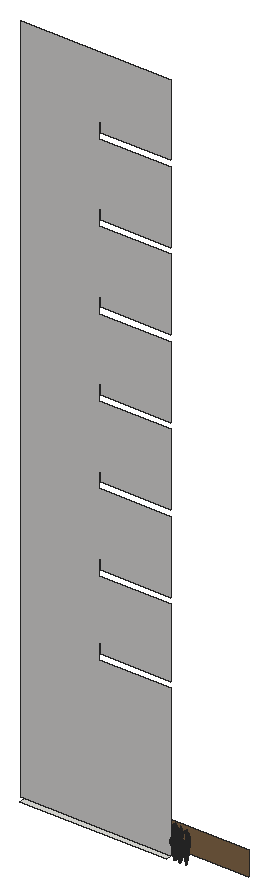
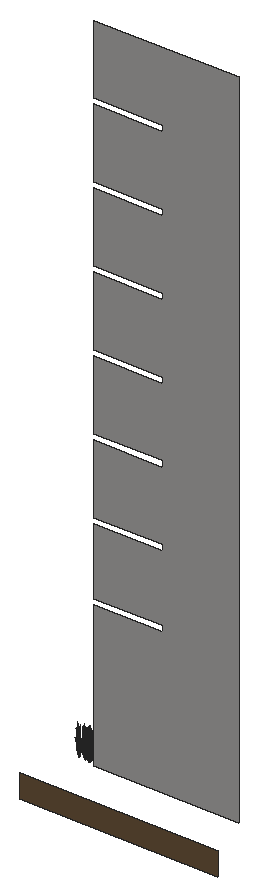
# SketchUp Ruby script. Lengths in inches.
U = 1.inch
M = Sketchup.active_model
def pt(a) = Geom::Point3d.new(a.map { |v| v * U })
def face(e, loops, mat)
  f = e.add_face(loops[0].map { |a| pt(a) })
  loops[1..].each { |l| e.add_face(l.map { |a| pt(a) }).erase! }
  f.material = f.back_material = mat if mat
  f
end
# faces: each face lists its corners as indices into pts; further lists are holes
def faces(e, pts, list, mat = nil) = list.each { |f| face(e, (f[0].is_a?(Array) ? f : [f]).map { |l| l.map { |i| pts[i] } }, mat) }
# xy, xz, yz: faces in a plane at the given z, y or x. An outline is a flat list of corners, or four numbers for a rectangle; further outlines are holes
def ring(l) = l.size == 4 ? [[l[0], l[1]], [l[2], l[1]], [l[2], l[3]], [l[0], l[3]]] : l.each_slice(2).to_a
def flat(e, list, mat, &to3) = list.each { |f| face(e, (f[0].is_a?(Array) ? f : [f]).map { |l| ring(l).map { |u, v| to3.(u, v) } }, mat) }
def xy(e, z, list, mat = nil) = flat(e, list, mat) { |x, y| [x, y, z] }
def xz(e, y, list, mat = nil) = flat(e, list, mat) { |x, z| [x, y, z] }
def yz(e, x, list, mat = nil) = flat(e, list, mat) { |y, z| [x, y, z] }
def lines(e, pts, list) = list.each { |a, b| e.add_line(pt(pts[a]), pt(pts[b])) }
# prism: a flat outline (further loops are holes) pulled along v
def prism(e, loops, v, mat = nil)
  f = face(e, loops, mat); d = Geom::Vector3d.new(v.map { |x| x * U })
  f.pushpull(f.normal.samedirection?(d) ? d.length : -d.length)
end
def box(e, o, s, mat = nil) = prism(e, [[o, [o[0] + s[0], o[1], o[2]], [o[0] + s[0], o[1] + s[1], o[2]], [o[0], o[1] + s[1], o[2]]]], [0, 0, s[2]], mat)
def at(x, y, z, deg = 0) = Geom::Transformation.translation(pt([x, y, z])) * Geom::Transformation.rotation(ORIGIN, Z_AXIS, deg.degrees)
def axes(o, x, y, z) = Geom::Transformation.new([*x, 0, *y, 0, *z, 0, *pt(o).to_a, 1])
def part(name) = M.definitions.add(name)
# library, detail: a bought-in or finely detailed component or shape, given as its bounding box
def library(name, o, s) = part(name).tap { |d| box(d.entities, o, s) }
def detail(e, o, s) = box(e.add_group.entities, o, s)
def put(e, d, t, mat = nil) = e.add_instance(d, t).tap { |i| i.material = mat if mat }
def group(e, t, mat = nil) = e.add_group.tap { |g| g.transformation = t; g.material = mat if mat }.entities
root = M.entities
M.materials.add("Carpet_01_1K").color = [196, 195, 193]
M.materials.add("LightPink_Translucent").color = [144, 107, 117]
M.materials["LightPink_Translucent"].alpha = 0.75
M.materials.add("Soil_03_1K").color = [122, 96, 67]
c1 = part("blade")
p = [[2.15,0.21,22],[0,0.17,0],[0.09,0.45,0],[2.18,0.31,22],[2.29,0.31,22],[0.38,0.45,0],
  [2.48,0.24,33],[2.49,0.24,33],[2.48,0.22,33]]
faces(c1.entities,p,[[0,1,2,3],[4,5,2,3],[6,3,4,7],[8,0,3,6]])
c2 = part("seeds")
p = [[0.3,-0.1,1.38],[-0.01,-0.03,1.59],[-0.01,-0.03,0.03],[0.14,-0.07,-0.07],[0.29,-0.03,3],[0.15,0.01,3.11]]
faces(c2.entities,p,[[0,1,2,3],[1,0,4,5]],"LightPink_Translucent")
c3 = part("blade with seeds")
put(c3.entities,c1,at(0,0,0))
put(c3.entities,c2,axes([2.4,0.25,30.99],[1.5799,-0.05474,1.17369],[-0.12525,1.92788,0.29478],[-0.07173,-0.02425,1.56792]))
xy(root,0,[[39.57,786.64,330.57,798.7]])
xz(root,798.7,[[30.57,0,30.57,1386,330.57,1386,330.57,1242,189.57,1242,189.57,1260,186.57,1260,186.57,1230,330.57,1230,330.57,1086,189.57,1086,189.57,1104,186.57,1104,186.57,1074,330.57,1074,330.57,930,189.57,930,189.57,948,186.57,948,186.57,918,330.57,918,330.57,774,189.57,774,189.57,791.9,186.57,791.9,186.57,762,330.57,762,330.57,618,189.57,618,189.57,636,186.57,636,186.57,606,330.57,606,330.57,462,189.57,462,189.57,480,186.57,480,186.57,450,330.57,450,330.57,312,189.57,312,189.57,330,186.57,330,186.57,300,330.57,300,330.57,0]],"Carpet_01_1K")
xz(root,890.67,[[0,-48,410.57,0]],"Soil_03_1K")
put(root,c3,axes([342.49,790.44,4.68],[-0.25628,0.30892,-0.51099],[-0.22444,-0.32634,-0.3958],[-0.13021,-0.047,0.97773]))
put(root,c3,axes([368.57,789.07,2.72],[0.38326,-0.02879,0.44739],[0.03466,0.47788,-0.21531],[-0.06861,0.04843,1.43643]))
put(root,c3,axes([368.8125,788.59,2.62],[0.32884,-0.136,0.1448],[0.11516,0.38837,-0.41347],[0,0.08547,1.26744]))
put(root,c3,axes([355.58,788.84,2.72],[0.17124,-0.42022,0.44739],[0.35581,0.20224,-0.21531],[0,0.09687,1.43643]))
put(root,c3,axes([341.92,790.85,2.77],[0.22533,-0.03337,1.1486],[-0.14293,0.29403,0.84392],[-0.11135,-0.04411,0.25299]))
put(root,c3,axes([368.23,789.3,2.21],[-0.38326,0.02879,-0.44739],[-0.03466,-0.47788,0.21531],[-0.06861,0.04843,1.43643]))
put(root,c3,axes([355.52,789.08,2.29],[0,0.53934,-0.05637],[-0.44133,0,0],[0,0.01695,1.79368]))
put(root,c3,axes([353.5,788.89,4.68],[-0.09562,0.42421,-0.51099],[-0.32782,-0.1454,-0.3958],[-0.13199,0.0389,0.97773]))
put(root,c3,axes([343.51,791.125,2.72],[-0.38326,0.02879,0.44739],[-0.03466,-0.47788,-0.21531],[0.06861,-0.04843,1.43643]))
put(root,c3,axes([355.55,788.7,2.21],[0.21202,0.39143,-0.44739],[-0.32115,0.27564,0.21531],[0.06861,0.04843,1.43643]))
put(root,c3,axes([356.99,790.36,3.93],[-0.06755,-0.39203,-0.03492],[0.31928,-0.09013,-0.15832],[0.06667,0.02485,0.52218]))
put(root,c3,axes([342.52,791.47,2.48],[0,0.46636,0.49651],[-0.39487,0,0],[0,-0.10622,1.57504]))
put(root,c3,axes([354.23,790.7,2.375],[-0.22066,0.46731,0],[-0.36918,-0.26061,-0.51607],[-0.08408,-0.05936,1.63711]))
put(root,c3,axes([345.29,791.58,4.68],[0.09562,-0.42421,-0.51099],[0.32782,0.1454,-0.3958],[0.13199,-0.0389,0.97773]))
put(root,c3,axes([344.77,789.85,2.375],[0.22066,-0.46731,0],[0.36918,0.26061,-0.51607],[0.08408,0.05936,1.63711]))
put(root,c3,axes([356.48,789.08,2.48],[0,-0.46636,0.49651],[0.39487,0,0],[0,0.10622,1.57504]))
put(root,c3,axes([342.17,790.77,3.875],[0.14639,-0.01056,1.71376],[-0.09712,0.45778,0.13857],[-0.20862,-0.02831,0.73262]))
put(root,c3,axes([368.52,789.95,2.2],[0.35581,0.20937,0],[-0.17124,0.43505,0],[0,0,1.74954]))
put(root,c3,axes([343.45,791.85,2.21],[-0.21202,-0.39143,-0.44739],[0.32115,-0.27564,0.21531],[-0.06861,-0.04843,1.43643]))
put(root,c3,axes([343.49,791.3,2.36],[0.15345,0.52148,0.45755],[-0.43845,0.18134,0.17955],[0.00536,-0.09582,1.58856]))
put(root,c3,axes([355.49,789.43,2.72],[0.38326,-0.02879,0.44739],[0.03466,0.47788,-0.21531],[-0.06861,0.04843,1.43643]))
put(root,c3,axes([355.73,788.9375,2.62],[0.32884,-0.136,0.1448],[0.11516,0.38837,-0.41347],[0,0.08547,1.26744]))
put(root,c3,axes([345.64,791.7,1.98],[-0.22732,0.05597,1.41583],[-0.03618,-0.44548,0.08104],[0.15921,-0.06743,0.80566]))
put(root,c3,axes([346.05,791.3,2.26],[-0.21881,-0.29821,-0.06488],[0.23965,-0.27324,-0.29416],[0.0679,-0.01924,0.97024]))
put(root,c3,axes([355.15,789.66,2.21],[-0.38326,0.02879,-0.44739],[-0.03466,-0.47788,0.21531],[-0.06861,0.04843,1.43643]))
put(root,c3,axes([368.66,790.41,2.19],[-0.21791,-0.46895,-0.05142],[0.36918,-0.26061,0.51607],[-0.09097,0.04465,1.6363]))
put(root,c3,axes([343.42,791.71,2.72],[-0.17124,0.42022,0.44739],[-0.35581,-0.20224,-0.21531],[0,-0.09687,1.43643]))
put(root,c3,axes([368.58,789.28,2.62],[0.26075,0.2802,0.1448],[-0.2175,0.31612,-0.41347],[-0.06054,0.04274,1.26744]))
put(root,c3,axes([344.05,791.34,2.21],[0,-0.53961,0],[0.44133,0,0],[0,0,1.79456]))
put(root,c3,axes([366.5625,788.75,3.875],[0.12246,-0.09864,1.71376],[0.1031,0.45582,0.13857],[-0.19225,0.10302,0.73262]))
put(root,c3,axes([356.96,789.89,2.59],[-0.085,-0.1147,1.43002],[0.1106,-0.37943,-0.30754],[0.17198,0.0514,0.61141]))
put(root,c3,axes([344.58,790.09,2.48],[-0.33032,-0.23318,0.49651],[0.19744,-0.41812,0],[0.07523,0.05311,1.57504]))
put(root,c3,axes([345.23,791.73,4.98],[0.31014,-0.20596,-0.71045],[0.17284,0.42397,0.08574],[0.14985,-0.04816,1.00501]))
put(root,c3,axes([355.4375,790.3,2.2],[0.35581,0.20937,0],[-0.17124,0.43505,0],[0,0,1.74954]))
put(root,c3,axes([343.26,792,2.06],[-0.36714,-0.07646,-0.62353],[0.07747,-0.47163,-0.16365],[-0.10956,-0.05715,1.37633]))
put(root,c3,axes([343.84,791,2.36],[-0.29264,0.42323,0.45755],[-0.34767,-0.3736,0.17955],[0.07055,-0.04224,1.58856]))
put(root,c3,axes([344.16,791.76,2.3],[-0.32829,-0.4014,-0.06131],[0.32849,-0.40164,0],[-0.01146,-0.01402,1.75571]))
put(root,c3,axes([355.58,790.77,2.19],[-0.21791,-0.46895,-0.05142],[0.36918,-0.26061,0.51607],[-0.09097,0.04465,1.6363]))
put(root,c3,axes([368.86,790.14,2.48],[0.33032,-0.23318,0.49651],[0.19744,0.41812,0],[-0.07523,0.05311,1.57504]))
put(root,c3,axes([355.5,789.63,2.62],[0.26075,0.2802,0.1448],[-0.2175,0.31612,-0.41347],[-0.06054,0.04274,1.26744]))
put(root,c3,axes([343.33,790.3,2.47],[-0.10196,0.46348,0.17642],[-0.3731,-0.13116,0.35086],[0.06445,-0.00226,1.60407]))
put(root,c3,axes([353.48,789.11,3.875],[0.12246,-0.09864,1.71376],[0.1031,0.45582,0.13857],[-0.19225,0.10302,0.73262]))
put(root,c3,axes([368.39,789.77,2.29],[0.15345,0.53576,-0.06012],[-0.43845,0.18773,0],[0.00536,0.01871,1.72173]))
put(root,c3,axes([368.56,790.35,2.03],[-0.32928,-0.11539,-0.30978],[0.08291,-0.40636,0.30978],[-0.06638,0.04686,1.38974]))
put(root,c3,axes([366.18,789.53,2.59],[0.12266,0.03828,1.43002],[0.07906,0.39104,-0.30754],[-0.16661,0.0732,0.61141]))
put(root,c3,axes([343.17,790.68,1.59],[-0.3474,0.18671,1.28929],[-0.11057,-0.53572,0.50096],[0.21332,0.00891,1.46642]))
put(root,c3,axes([344.11,790.82,2.62],[0.06809,-0.4162,0.1448],[0.33266,0.07225,-0.41347],[0.06054,0.04274,1.26744]))
put(root,c3,axes([343.53,791.81,2.36],[0.44609,0.09826,0.45755],[-0.09078,0.55493,0.17955],[-0.06519,-0.05359,1.58856]))
put(root,c3,axes([369.66,789.07,2.2],[-0.44111,-0.00373,-0.04976],[0,-0.52122,0.49943],[-0.01386,0.11865,1.58352]))
put(root,c3,axes([345.89,791.41,1.49],[-0.01845,-0.0708,1.76342],[0.12793,-0.41416,-0.26939],[0.12905,-0.00596,0.30037]))
put(root,c3,axes([356.18,790.12,4.98],[0.35281,0.01123,-0.71045],[-0.0237,0.47284,0.08574],[0.14947,0.0499,1.00501]))
put(root,c3,axes([342.08,791.33,1.49],[0.00895,0.0735,1.76342],[-0.18044,0.38382,-0.26939],[-0.12817,-0.01935,0.30037]))
put(root,c3,axes([343.97,790.93,2.72],[-0.21202,-0.39143,0.44739],[0.32115,-0.27564,-0.21531],[0.06861,0.04843,1.43643]))
put(root,c3,axes([365.93,790.35,2.77],[0.14709,-0.21136,1.1486],[0.05804,0.3346,0.84392],[-0.1063,0.05991,0.25299]))
put(root,c3,axes([369.5625,789.15,2.03],[-0.24637,0.29097,-0.30978],[-0.24637,-0.29097,0.30978],[0,0.09372,1.38974]))
put(root,c3,axes([355.78,790.5,2.48],[0.33032,-0.23318,0.49651],[0.19744,0.41812,0],[-0.07523,0.05311,1.57504]))
put(root,c3,axes([368.5,789.17,2.67],[0.04113,0.53214,-0.29095],[-0.42835,0.03218,-0.50002],[-0.07543,0.07088,1.59708]))
put(root,c3,axes([342.87,792.72,2.03],[-0.08291,-0.40636,-0.30978],[0.32928,-0.11539,0.30978],[-0.06638,-0.04686,1.38974]))
put(root,c3,axes([355.31,790.13,2.29],[0.15345,0.53576,-0.06012],[-0.43845,0.18773,0],[0.00536,0.01871,1.72173]))
put(root,c3,axes([368.66,788.97,2.21],[-0.17124,0.42022,-0.44739],[-0.35581,-0.20224,0.21531],[0,0.09687,1.43643]))
put(root,c3,axes([366.48,789.43,4.53],[-0.30722,0.06665,-0.35414],[-0.08112,-0.381,0.4572],[-0.08804,0.10234,0.87481]))
put(root,c3,axes([355.48,790.71,2.03],[-0.32928,-0.11539,-0.30978],[0.08291,-0.40636,0.30978],[-0.06638,0.04686,1.38974]))
put(root,c3,axes([353.1,789.88,2.59],[0.12266,0.03828,1.43002],[0.07906,0.39104,-0.30754],[-0.16661,0.0732,0.61141]))
put(root,c3,axes([343.29,792.69,2.47],[0.37926,-0.12378,0.17642],[0.09365,0.46065,0.35086],[-0.03382,-0.06712,1.60407]))
put(root,c3,axes([344.07,790.95,2.67],[0.35635,-0.30962,-0.29095],[0.23697,0.43749,-0.50002],[0.08792,0.04443,1.59708]))
put(root,c3,axes([345.49,791.77,4.53],[0.29332,0.1301,-0.35414],[-0.08555,0.37955,0.4572],[0.11809,-0.0348,0.87481]))
put(root,c3,axes([356.75,789.16,2.375],[0.44133,0,0],[0,0.52122,-0.51607],[0,0.11871,1.63711]))
put(root,c3,axes([356.58,789.42,2.2],[-0.44111,-0.00373,-0.04976],[0,-0.52122,0.49943],[-0.01386,0.11865,1.58352]))
put(root,c3,axes([355.62,788.97,2.67],[0.39748,0.22252,-0.29095],[-0.19139,0.46966,-0.50002],[0.01249,0.11531,1.59708]))
put(root,c3,axes([342.78,792.89,2.02],[-0.33032,-0.23318,-0.49651],[0.19744,-0.41812,0],[-0.07523,-0.05311,1.57504]))
put(root,c3,axes([344.97,790.13,2.02],[0.33032,0.23318,-0.49651],[-0.19744,0.41812,0],[0.07523,0.05311,1.57504]))
put(root,c3,axes([342.04,791.17,4.53],[-0.29332,-0.1301,-0.35414],[0.08555,-0.37955,0.4572],[-0.11809,0.0348,0.87481]))
put(root,c3,axes([352.85,790.7,2.77],[0.14709,-0.21136,1.1486],[0.05804,0.3346,0.84392],[-0.1063,0.05991,0.25299]))
put(root,c3,axes([356.39,790.3125,4.53],[0.20082,0.29199,-0.35414],[-0.2293,0.2764,0.4572],[0.1165,0.04206,0.87481]))
put(root,c3,axes([356.48,789.5,2.03],[-0.24637,0.29097,-0.30978],[-0.24637,-0.29097,0.30978],[0,0.09372,1.38974]))
put(root,c3,axes([344.35,791.46,2.21],[0.39487,0,0],[0,0.48281,0],[0,0,1.78407]))
put(root,c3,axes([355.42,789.53,2.67],[0.04113,0.53214,-0.29095],[-0.42835,0.03218,-0.50002],[-0.07543,0.07088,1.59708]))
put(root,c3,axes([368.24,789.58,2.06],[-0.23773,0.35053,-0.62353],[-0.29532,-0.31785,-0.16365],[-0.09526,0.08744,1.37633]))
put(root,c3,axes([343.68,792.07,2.67],[-0.35635,0.30962,-0.29095],[-0.23697,-0.43749,-0.50002],[-0.08792,-0.04443,1.59708]))
put(root,c3,axes([344.46,790.33,2.47],[-0.37926,0.12378,0.17642],[-0.09365,-0.46065,0.35086],[0.03382,0.06712,1.60407]))
put(root,c3,axes([355.58,789.32,2.21],[-0.17124,0.42022,-0.44739],[-0.35581,-0.20224,0.21531],[0,0.09687,1.43643]))
put(root,c3,axes([353.4,789.79,4.53],[-0.30722,0.06665,-0.35414],[-0.08112,-0.381,0.4572],[-0.08804,0.10234,0.87481]))
put(root,c3,axes([368.67,790.17,2.33],[0.44186,0.15158,0.30756],[-0.11054,0.54181,-0.36492],[-0.07313,0.06781,1.64885]))
put(root,c3,axes([344.69,791.3,3.875],[-0.14639,0.01056,1.71376],[0.09712,-0.45778,0.13857],[0.20862,0.02831,0.73262]))
put(root,c3,axes([368.64,790.54,2.02],[-0.33032,0.23318,-0.49651],[-0.19744,-0.41812,0],[-0.07523,0.05311,1.57504]))
put(root,c3,axes([344.88,790.31,2.03],[0.08291,0.40636,-0.30978],[-0.32928,0.11539,0.30978],[0.06638,0.04686,1.38974]))
put(root,c3,axes([344.22,791.22,2.38],[-0.44609,-0.09826,0.49198],[0.09078,-0.55493,0.19306],[0.06519,0.05359,1.70813]))
put(root,c3,axes([355.16,789.93,2.06],[-0.23773,0.35053,-0.62353],[-0.29532,-0.31785,-0.16365],[-0.09526,0.08744,1.37633]))
put(root,c3,axes([343.86,792.59,2.2],[-0.11516,-0.40207,0],[0.32884,-0.1408,0],[0,0,1.54371]))
put(root,c3,axes([343.64,792.2,2.62],[-0.06809,0.4162,0.1448],[-0.33266,-0.07225,-0.41347],[-0.06054,-0.04274,1.26744]))
put(root,c3,axes([344.29,792.53,2.18],[0.37054,-0.15823,-0.19198],[0.1302,0.45581,0.00008],[0.0409,-0.01749,1.73897]))
put(root,c3,axes([355.59,790.53,2.33],[0.44186,0.15158,0.30756],[-0.11054,0.54181,-0.36492],[-0.07313,0.06781,1.64885]))
put(root,c3,axes([355.56,790.89,2.02],[-0.33032,0.23318,-0.49651],[-0.19744,-0.41812,0],[-0.07523,0.05311,1.57504]))
put(root,c3,axes([356.65,789.51,2.02],[0,0.46636,-0.49651],[-0.39487,0,0],[0,0.10622,1.57504]))
put(root,c3,axes([344.42,792.72,2.47],[0.10196,-0.46348,0.17642],[0.3731,0.13116,0.35086],[-0.06445,0.00226,1.60407]))
put(root,c3,axes([367.01,789.06,3.875],[0.08815,-0.14329,1.71376],[0.22258,0.38678,0.13857],[-0.15267,0.17614,0.73262]))
put(root,c3,axes([355.67,789.5625,3.875],[-0.1311,-0.08035,1.71376],[0.27131,-0.33708,0.13857],[0.16909,0.15206,0.73262]))
put(root,c3,axes([344.34,791.67,2.21],[0.24637,0.30123,0],[-0.24637,0.30123,0],[0,0,1.69266]))
put(root,c3,axes([366.73,789.48,4.68],[0.09067,0.42583,-0.51099],[-0.34336,0.07449,-0.3958],[-0.0984,0.11438,0.97773]))
put(root,c3,axes([342.9375,791.1,3.34],[0.10032,-0.06746,1.77064],[0.0346,0.47103,0.13857],[-0.2173,0.0625,0.63284]))
put(root,c3,axes([345,791.54,2.47],[-0.2773,-0.3397,0.17642],[0.27945,-0.32949,0.35086],[-0.03063,0.06937,1.60407]))
put(root,c3,axes([344.49,791.02,2.06],[0.36714,0.07646,-0.62353],[-0.07747,0.47163,-0.16365],[0.10956,0.05715,1.37633]))
put(root,c3,axes([368.94,790.46,2.375],[0.22066,0.46731,0],[-0.36918,0.26061,-0.51607],[-0.08408,0.05936,1.63711]))
put(root,c3,axes([346.11,791.85,2.77],[-0.21807,0.07699,1.1486],[0.10265,-0.31819,0.84392],[0.11568,0.02177,0.25299]))
put(root,c3,axes([356.15,790.48,2.77],[-0.19872,-0.13409,1.1486],[0.2566,-0.13625,0.84392],[0.06921,0.11541,0.25299]))
put(root,c3,axes([368.75,788.61,2.84],[-0.00964,-0.43909,1.41272],[0.43635,0.11382,0.59816],[-0.1032,0.24027,1.3335]))
put(root,c3,axes([368.86,789.09,2.09],[0.12941,0.42699,-0.69212],[-0.37279,0.15378,-0.18165],[0.0143,0.14459,1.52773]))
put(root,c3,axes([343.78,792.77,2.2],[-0.35581,-0.20937,0],[0.17124,-0.43505,0],[0,0,1.62707]))
put(root,c3,axes([344.08,792.21,2.46],[-0.34464,-0.37536,-0.25192],[0.29,-0.42149,0.5513],[-0.0928,0.04391,1.68216]))
put(root,c3,axes([366.3125,790.56,1.49],[0.04734,0.04659,1.76342],[0.08027,0.4317,-0.26939],[-0.10492,0.09206,0.30037]))
put(root,c3,axes([343.17,792.93,2.48],[0.33032,0.23318,0.49651],[-0.19744,0.41812,0],[-0.07523,-0.05311,1.57504]))
put(root,c3,axes([353.93,789.41,3.875],[0.08815,-0.14329,1.71376],[0.22258,0.38678,0.13857],[-0.15267,0.17614,0.73262]))
put(root,c3,axes([344.33,791.32,2.72],[0.17124,-0.42022,0.44739],[0.35581,0.20224,-0.21531],[0,0.09687,1.43643]))
put(root,c3,axes([353.65,789.83,4.68],[0.09067,0.42583,-0.51099],[-0.34336,0.07449,-0.3958],[-0.0984,0.11438,0.97773]))
put(root,c3,axes([355.86,790.82,2.375],[0.22066,0.46731,0],[-0.36918,0.26061,-0.51607],[-0.08408,0.05936,1.63711]))
put(root,c3,axes([344.27,791.56,2.29],[0,0.53934,-0.05637],[-0.44133,0,0],[0,0.01695,1.79368]))
put(root,c3,axes([342.24,791.36,4.68],[-0.09562,0.42421,-0.51099],[-0.32782,-0.1454,-0.3958],[-0.13199,0.0389,0.97773]))
put(root,c3,axes([344.3,791.17,2.21],[0.21202,0.39143,-0.44739],[-0.32115,0.27564,0.21531],[0.06861,0.04843,1.43643]))
put(root,c3,axes([345.73,792.83,3.93],[-0.06755,-0.39203,-0.03492],[0.31928,-0.09013,-0.15832],[0.06667,0.02485,0.52218]))
put(root,c3,axes([356.21,790.98,1.49],[0.02571,-0.06733,1.76342],[0.32373,-0.19829,-0.26939],[0.09815,0.10263,0.30037]))
put(root,c3,axes([355.67,788.97,2.84],[-0.00964,-0.43909,1.41272],[0.43635,0.11382,0.59816],[-0.1032,0.24027,1.3335]))
put(root,c3,axes([355.78,789.45,2.09],[0.12941,0.42699,-0.69212],[-0.37279,0.15378,-0.18165],[0.0143,0.14459,1.52773]))
put(root,c3,axes([342.98,793.17,2.375],[-0.22066,0.46731,0],[-0.36918,-0.26061,-0.51607],[-0.08408,-0.05936,1.63711]))
put(root,c3,axes([353.23,790.92,1.49],[0.04734,0.04659,1.76342],[0.08027,0.4317,-0.26939],[-0.10492,0.09206,0.30037]))
put(root,c3,axes([355.7,790.66,4.68],[0.34827,-0.11086,-0.51099],[0.06092,0.41983,-0.3958],[0.09354,0.12031,0.97773]))
put(root,c3,axes([345.23,791.55,2.48],[0,-0.46636,0.49651],[0.39487,0,0],[0,0.10622,1.57504]))
put(root,c3,axes([344.24,791.9,2.72],[0.38326,-0.02879,0.44739],[0.03466,0.47788,-0.21531],[-0.06861,0.04843,1.43643]))
put(root,c3,axes([344.48,791.41,2.62],[0.32884,-0.136,0.1448],[0.11516,0.38837,-0.41347],[0,0.08547,1.26744]))
put(root,c3,axes([343.9,792.13,2.21],[-0.38326,0.02879,-0.44739],[-0.03466,-0.47788,0.21531],[-0.06861,0.04843,1.43643]))
put(root,c3,axes([366.95,789.41,3.875],[0.06572,-0.16029,1.71376],[0.27569,0.33172,0.13857],[-0.12437,0.20675,0.73262]))
put(root,c3,axes([356.18,791.09,2.67],[-0.22633,-0.01463,1.0506],[0.14947,-0.31064,0.58006],[0.08941,0.11036,0.8241]))
put(root,c3,axes([345.7,792.36,2.59],[-0.085,-0.1147,1.43002],[0.1106,-0.37943,-0.30754],[0.17198,0.0514,0.61141]))
put(root,c3,axes([344.18,792.78,2.2],[0.35581,0.20937,0],[-0.17124,0.43505,0],[0,0,1.74954]))
put(root,c3,axes([367.02,790.32,4.53],[-0.23881,0.24554,-0.35414],[-0.22606,-0.28036,0.4572],[-0.0344,0.14245,0.87481]))
put(root,c3,axes([367.17,791.27,2.77],[-0.00913,-0.2773,1.1486],[0.22824,0.19778,0.84392],[-0.04489,0.13217,0.25299]))
put(root,c3,axes([344.33,793.24,2.19],[-0.21791,-0.46895,-0.05142],[0.36918,-0.26061,0.51607],[-0.09097,0.04465,1.6363]))
put(root,c3,axes([353.87,789.77,3.875],[0.06572,-0.16029,1.71376],[0.27569,0.33172,0.13857],[-0.12437,0.20675,0.73262]))
put(root,c3,axes([344.25,792.1,2.62],[0.26075,0.2802,0.1448],[-0.2175,0.31612,-0.41347],[-0.06054,0.04274,1.26744]))
put(root,c3,axes([342.23,791.58,3.875],[0.12246,-0.09864,1.71376],[0.1031,0.45582,0.13857],[-0.19225,0.10302,0.73262]))
put(root,c3,axes([355.44,790.34,2.59],[0.00623,-0.15459,1.43002],[0.29764,-0.17268,-0.30754],[0.09188,0.18503,0.61141]))
put(root,c3,axes([367.77,790.61,1.49],[0.05712,-0.02538,1.76342],[0.34359,0.13968,-0.26939],[0.01005,0.15742,0.30037]))
put(root,c3,axes([353.94,790.67,4.53],[-0.23881,0.24554,-0.35414],[-0.22606,-0.28036,0.4572],[-0.0344,0.14245,0.87481]))
put(root,c3,axes([367.26,790.2,5],[0.25266,0.31335,-0.5672],[-0.2669,0.27442,-0.43934],[-0.03844,0.15921,1.08528]))
put(root,c3,axes([344.92,792.59,4.98],[0.35281,0.01123,-0.71045],[-0.0237,0.47284,0.08574],[0.14947,0.0499,1.00501]))
put(root,c3,axes([354.09,791.625,2.77],[-0.00913,-0.2773,1.1486],[0.22824,0.19778,0.84392],[-0.04489,0.13217,0.25299]))
put(root,c3,axes([366.99,790.67,2.82],[0.32063,-0.08258,0.06507],[0.07371,0.33271,-0.86304],[-0.02033,0.16842,0.7736]))
put(root,c3,axes([368.01,790.5,4.68],[0.34695,0.11691,-0.51099],[-0.11892,0.40083,-0.3958],[0.03181,0.16138,0.97773]))
put(root,c3,axes([344.53,792.97,2.48],[0.33032,-0.23318,0.49651],[0.19744,0.41812,0],[-0.07523,0.05311,1.57504]))
put(root,c3,axes([344.06,792.6,2.29],[0.15345,0.53576,-0.06012],[-0.43845,0.18773,0],[0.00536,0.01871,1.72173]))
put(root,c3,axes([344.23,793.18,2.03],[-0.32928,-0.11539,-0.30978],[0.08291,-0.40636,0.30978],[-0.06638,0.04686,1.38974]))
put(root,c3,axes([354.7,790.96,1.49],[0.05712,-0.02538,1.76342],[0.34359,0.13968,-0.26939],[0.01005,0.15742,0.30037]))
put(root,c3,axes([341.85,792.36,2.59],[0.12266,0.03828,1.43002],[0.07906,0.39104,-0.30754],[-0.16661,0.0732,0.61141]))
put(root,c3,axes([367.85,790.75,4.53],[-0.1064,0.35863,-0.35414],[-0.31043,-0.1046,0.4572],[0.02846,0.14439,0.87481]))
put(root,c3,axes([345.5,791.63,2.375],[0.44133,0,0],[0,0.52122,-0.51607],[0,0.11871,1.63711]))
put(root,c3,axes([345.32,791.9,2.2],[-0.44111,-0.00373,-0.04976],[0,-0.52122,0.49943],[-0.01386,0.11865,1.58352]))
put(root,c3,axes([354.18,790.55,5],[0.25266,0.31335,-0.5672],[-0.2669,0.27442,-0.43934],[-0.03844,0.15921,1.08528]))
put(root,c3,axes([344.37,791.44,2.67],[0.39748,0.22252,-0.29095],[-0.19139,0.46966,-0.50002],[0.01249,0.11531,1.59708]))
put(root,c3,axes([367.18,790.06,5.34],[-0.00918,0.43138,-0.7886],[-0.38672,-0.02897,0.09517],[-0.04081,0.18275,1.11556]))
put(root,c3,axes([341.6,793.17,2.77],[0.14709,-0.21136,1.1486],[0.05804,0.3346,0.84392],[-0.1063,0.05991,0.25299]))
put(root,c3,axes([353.91,791.02,2.82],[0.32063,-0.08258,0.06507],[0.07371,0.33271,-0.86304],[-0.02033,0.16842,0.7736]))
put(root,c3,axes([345.14,792.78,4.53],[0.20082,0.29199,-0.35414],[-0.2293,0.2764,0.4572],[0.1165,0.04206,0.87481]))
put(root,c3,axes([345.23,791.97,2.03],[-0.24637,0.29097,-0.30978],[-0.24637,-0.29097,0.30978],[0,0.09372,1.38974]))
put(root,c3,axes([354.93,790.86,4.68],[0.34695,0.11691,-0.51099],[-0.11892,0.40083,-0.3958],[0.03181,0.16138,0.97773]))
put(root,c3,axes([355.125,790.03,3.875],[-0.08068,-0.14973,1.71376],[0.3728,-0.12606,0.13857],[0.08426,0.23506,0.73262]))
put(root,c3,axes([344.17,792,2.67],[0.04113,0.53214,-0.29095],[-0.42835,0.03218,-0.50002],[-0.07543,0.07088,1.59708]))
put(root,c3,axes([344.33,791.79,2.21],[-0.17124,0.42022,-0.44739],[-0.35581,-0.20224,0.21531],[0,0.09687,1.43643]))
put(root,c3,axes([342.15,792.26,4.53],[-0.30722,0.06665,-0.35414],[-0.08112,-0.381,0.4572],[-0.08804,0.10234,0.87481]))
put(root,c3,axes([367.55,789.75,3.875],[-0.00864,-0.17899,1.71376],[0.37441,0.11874,0.13857],[-0.02316,0.25508,0.73262]))
put(root,c3,axes([354.77,791.1,4.53],[-0.1064,0.35863,-0.35414],[-0.31043,-0.1046,0.4572],[0.02846,0.14439,0.87481]))
put(root,c3,axes([367.88,790.43,4.98],[0.16845,0.3792,-0.71045],[-0.34676,0.21133,0.08574],[0.03939,0.18322,1.00501]))
put(root,c3,axes([354.1,790.41,5.34],[-0.00918,0.43138,-0.7886],[-0.38672,-0.02897,0.09517],[-0.04081,0.18275,1.11556]))
put(root,c3,axes([343.91,792.41,2.06],[-0.23773,0.35053,-0.62353],[-0.29532,-0.31785,-0.16365],[-0.09526,0.08744,1.37633]))
put(root,c3,axes([366.91,791.02,2.59],[0.11138,-0.07357,1.43002],[0.27499,0.22183,-0.30754],[-0.08185,0.19194,0.61141]))
put(root,c3,axes([354.47,790.1,3.875],[-0.00864,-0.17899,1.71376],[0.37441,0.11874,0.13857],[-0.02316,0.25508,0.73262]))
put(root,c3,axes([344.34,793,2.33],[0.44186,0.15158,0.30756],[-0.11054,0.54181,-0.36492],[-0.07313,0.06781,1.64885]))
put(root,c3,axes([344.3,793.36,2.02],[-0.33032,0.23318,-0.49651],[-0.19744,-0.41812,0],[-0.07523,0.05311,1.57504]))
put(root,c3,axes([345.4,791.98,2.02],[0,0.46636,-0.49651],[-0.39487,0,0],[0,0.10622,1.57504]))
put(root,c3,axes([344.41,792.04,3.875],[-0.1311,-0.08035,1.71376],[0.27131,-0.33708,0.13857],[0.16909,0.15206,0.73262]))
put(root,c3,axes([354.8,790.78,4.98],[0.16845,0.3792,-0.71045],[-0.34676,0.21133,0.08574],[0.03939,0.18322,1.00501]))
put(root,c3,axes([353.83,791.38,2.59],[0.11138,-0.07357,1.43002],[0.27499,0.22183,-0.30754],[-0.08185,0.19194,0.61141]))
put(root,c3,axes([344.9,792.95,2.77],[-0.19872,-0.13409,1.1486],[0.2566,-0.13625,0.84392],[0.06921,0.11541,0.25299]))
put(root,c3,axes([342.68,791.89,3.875],[0.08815,-0.14329,1.71376],[0.22258,0.38678,0.13857],[-0.15267,0.17614,0.73262]))
put(root,c3,axes([367.05,790.66,3.36],[0.00775,-0.24075,1.54345],[0.34877,0.12716,0.21329],[-0.03022,0.25658,0.72882]))
put(root,c3,axes([342.4,792.31,4.68],[0.09067,0.42583,-0.51099],[-0.34336,0.07449,-0.3958],[-0.0984,0.11438,0.97773]))
put(root,c3,axes([344.6,793.29,2.375],[0.22066,0.46731,0],[-0.36918,0.26061,-0.51607],[-0.08408,0.05936,1.63711]))
put(root,c3,axes([344.96,793.45,1.49],[0.02571,-0.06733,1.76342],[0.32373,-0.19829,-0.26939],[0.09815,0.10263,0.30037]))
put(root,c3,axes([344.42,791.44,2.84],[-0.00964,-0.43909,1.41272],[0.43635,0.11382,0.59816],[-0.1032,0.24027,1.3335]))
put(root,c3,axes([344.53,791.92,2.09],[0.12941,0.42699,-0.69212],[-0.37279,0.15378,-0.18165],[0.0143,0.14459,1.52773]))
put(root,c3,axes([341.98,793.39,1.49],[0.04734,0.04659,1.76342],[0.08027,0.4317,-0.26939],[-0.10492,0.09206,0.30037]))
put(root,c3,axes([344.45,793.14,4.68],[0.34827,-0.11086,-0.51099],[0.06092,0.41983,-0.3958],[0.09354,0.12031,0.97773]))
put(root,c3,axes([353.97,791.02,3.36],[0.00775,-0.24075,1.54345],[0.34877,0.12716,0.21329],[-0.03022,0.25658,0.72882]))
put(root,c3,axes([344.93,793.5625,2.67],[-0.22633,-0.01463,1.0506],[0.14947,-0.31064,0.58006],[0.08941,0.11036,0.8241]))
put(root,c3,axes([342.61,792.24,3.875],[0.06572,-0.16029,1.71376],[0.27569,0.33172,0.13857],[-0.12437,0.20675,0.73262]))
put(root,c3,axes([344.19,792.81,2.59],[0.00623,-0.15459,1.43002],[0.29764,-0.17268,-0.30754],[0.09188,0.18503,0.61141]))
put(root,c3,axes([342.69,793.14,4.53],[-0.23881,0.24554,-0.35414],[-0.22606,-0.28036,0.4572],[-0.0344,0.14245,0.87481]))
put(root,c3,axes([342.84,794.1,2.77],[-0.00913,-0.2773,1.1486],[0.22824,0.19778,0.84392],[-0.04489,0.13217,0.25299]))
put(root,c3,axes([343.44,793.43,1.49],[0.05712,-0.02538,1.76342],[0.34359,0.13968,-0.26939],[0.01005,0.15742,0.30037]))
put(root,c3,axes([342.93,793.03,5],[0.25266,0.31335,-0.5672],[-0.2669,0.27442,-0.43934],[-0.03844,0.15921,1.08528]))
put(root,c3,axes([342.65,793.5,2.82],[0.32063,-0.08258,0.06507],[0.07371,0.33271,-0.86304],[-0.02033,0.16842,0.7736]))
put(root,c3,axes([343.68,793.33,4.68],[0.34695,0.11691,-0.51099],[-0.11892,0.40083,-0.3958],[0.03181,0.16138,0.97773]))
put(root,c3,axes([343.875,792.5,3.875],[-0.08068,-0.14973,1.71376],[0.3728,-0.12606,0.13857],[0.08426,0.23506,0.73262]))
put(root,c3,axes([343.52,793.58,4.53],[-0.1064,0.35863,-0.35414],[-0.31043,-0.1046,0.4572],[0.02846,0.14439,0.87481]))
put(root,c3,axes([342.85,792.88,5.34],[-0.00918,0.43138,-0.7886],[-0.38672,-0.02897,0.09517],[-0.04081,0.18275,1.11556]))
put(root,c3,axes([343.22,792.58,3.875],[-0.00864,-0.17899,1.71376],[0.37441,0.11874,0.13857],[-0.02316,0.25508,0.73262]))
put(root,c3,axes([343.55,793.25,4.98],[0.16845,0.3792,-0.71045],[-0.34676,0.21133,0.08574],[0.03939,0.18322,1.00501]))
put(root,c3,axes([342.58,793.85,2.59],[0.11138,-0.07357,1.43002],[0.27499,0.22183,-0.30754],[-0.08185,0.19194,0.61141]))
put(root,c3,axes([342.72,793.49,3.36],[0.00775,-0.24075,1.54345],[0.34877,0.12716,0.21329],[-0.03022,0.25658,0.72882]))
